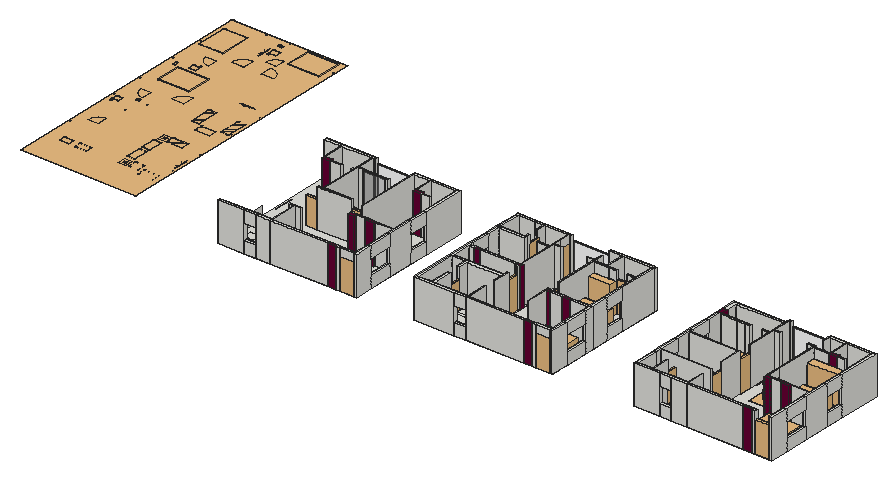
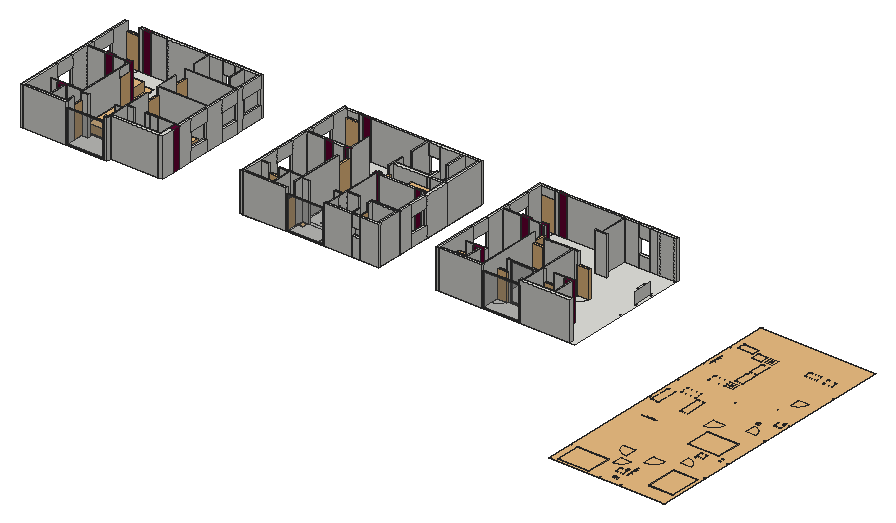
# SketchUp Ruby script. Lengths in inches.
U = 1.inch
M = Sketchup.active_model
def pt(a) = Geom::Point3d.new(a.map { |v| v * U })
def face(e, loops, mat)
  f = e.add_face(loops[0].map { |a| pt(a) })
  loops[1..].each { |l| e.add_face(l.map { |a| pt(a) }).erase! }
  f.material = f.back_material = mat if mat
  f
end
# faces: each face lists its corners as indices into pts; further lists are holes
def faces(e, pts, list, mat = nil) = list.each { |f| face(e, (f[0].is_a?(Array) ? f : [f]).map { |l| l.map { |i| pts[i] } }, mat) }
# xy, xz, yz: faces in a plane at the given z, y or x. An outline is a flat list of corners, or four numbers for a rectangle; further outlines are holes
def ring(l) = l.size == 4 ? [[l[0], l[1]], [l[2], l[1]], [l[2], l[3]], [l[0], l[3]]] : l.each_slice(2).to_a
def flat(e, list, mat, &to3) = list.each { |f| face(e, (f[0].is_a?(Array) ? f : [f]).map { |l| ring(l).map { |u, v| to3.(u, v) } }, mat) }
def xy(e, z, list, mat = nil) = flat(e, list, mat) { |x, y| [x, y, z] }
def xz(e, y, list, mat = nil) = flat(e, list, mat) { |x, z| [x, y, z] }
def yz(e, x, list, mat = nil) = flat(e, list, mat) { |y, z| [x, y, z] }
def lines(e, pts, list) = list.each { |a, b| e.add_line(pt(pts[a]), pt(pts[b])) }
# prism: a flat outline (further loops are holes) pulled along v
def prism(e, loops, v, mat = nil)
  f = face(e, loops, mat); d = Geom::Vector3d.new(v.map { |x| x * U })
  f.pushpull(f.normal.samedirection?(d) ? d.length : -d.length)
end
def box(e, o, s, mat = nil) = prism(e, [[o, [o[0] + s[0], o[1], o[2]], [o[0] + s[0], o[1] + s[1], o[2]], [o[0], o[1] + s[1], o[2]]]], [0, 0, s[2]], mat)
def at(x, y, z, deg = 0) = Geom::Transformation.translation(pt([x, y, z])) * Geom::Transformation.rotation(ORIGIN, Z_AXIS, deg.degrees)
def axes(o, x, y, z) = Geom::Transformation.new([*x, 0, *y, 0, *z, 0, *pt(o).to_a, 1])
def part(name) = M.definitions.add(name)
# library, detail: a bought-in or finely detailed component or shape, given as its bounding box
def library(name, o, s) = part(name).tap { |d| box(d.entities, o, s) }
def detail(e, o, s) = box(e.add_group.entities, o, s)
def put(e, d, t, mat = nil) = e.add_instance(d, t).tap { |i| i.material = mat if mat }
def group(e, t, mat = nil) = e.add_group.tap { |g| g.transformation = t; g.material = mat if mat }.entities
root = M.entities
M.materials.add("L08_Velvet_Rose").color = [102, 0, 51]
M.materials.add("[Color M07]").color = [58, 58, 58]
M.materials.add("[Translucent Glass Gray]3").color = [128, 128, 128]
M.materials["[Translucent Glass Gray]3"].alpha = 0.3
c1 = library("CS300DRT",[0,0,0],[27.18,17.85,30.31])
c2 = library("PINTU+6+YA",[0,-0.6875,0],[35.83,8.07,80.71])
c3 = library("T4592TW1\#2",[64.87,43.1,3.9375],[29.53,8.27,84.64])
c4 = part("WINDOW (1)")
xy(c4.entities,0,[[0,0,59.06,1.97]],"[Color M07]")
xy(c4.entities,1.97,[[1.97,0,57.09,0.98],[1.97,0.98,57.09,1.97]],"[Color M07]")
xy(c4.entities,104.33,[[1.97,0,57.09,0.98],[1.97,0.98,57.09,1.97]],"[Color M07]")
xy(c4.entities,106.3,[[0,0,59.06,1.97]],"[Color M07]")
xz(c4.entities,0,[[[0,0,59.06,106.3],[1.97,1.97,57.09,104.33]]],"[Color M07]")
xz(c4.entities,0.98,[[1.97,1.97,57.09,104.33]],"[Translucent Glass Gray]3")
xz(c4.entities,1.97,[[[0,0,59.06,106.3],[1.97,1.97,57.09,104.33]]],"[Color M07]")
yz(c4.entities,0,[[0,0,1.97,106.3]],"[Color M07]")
yz(c4.entities,1.97,[[0,1.97,0.98,104.33],[0.98,1.97,1.97,104.33]],"[Color M07]")
yz(c4.entities,57.09,[[0,1.97,0.98,104.33],[0.98,1.97,1.97,104.33]],"[Color M07]")
yz(c4.entities,59.06,[[0,0,1.97,106.3]],"[Color M07]")
c5 = part("A$C31921E4A")
p = [[-49.5,1.5,0],[-206.5,1.5,0],[-206.5,10.5,0],[-49.5,10.5,0],[-54.5,119.5,0],[-215.5,119.5,0],
  [-215.5,130.5,0],[-54.5,130.5,0],[206.5,140.5,0],[-54.5,140.5,0],[-54.5,129.5,0],[206.5,129.5,0],
  [215.5,193.5,0],[-215.5,193.5,0],[-215.5,202.5,0],[215.5,202.5,0],[215.5,-202.5,0],[-215.5,-202.5,0],
  [-215.5,-193.5,0],[215.5,-193.5,0],[-215.5,201.5,0],[-206.5,201.5,0],[-206.5,-193.5,0],[-54,201.5,0],
  [-45,201.5,0],[-45,-193.5,0],[-54,-193.5,0],[69,201.5,0],[82.5,201.5,0],[82.5,-54.5,0],
  [69,-54.5,0],[206.5,201.5,0],[215.5,201.5,0],[206.5,-193.5,0],[-206.5,-104.5,0],[-13.5,-104.5,0],
  [-13.5,-113.5,0],[-206.5,-113.5,0],[73.5,-45.5,0],[215.5,-45.5,0],[215.5,-54.5,0],[73.5,-54.5,0]]
lines(c5.entities,p,[[0,1],[1,2],[2,3],[4,5],[5,6],[6,7],[7,4],[8,9],[9,10],[10,11],[11,8],[12,13],
  [13,14],[14,15],[15,12],[16,17],[17,18],[18,19],[19,16],[20,21],[21,22],[22,18],[18,20],[23,24],
  [24,25],[25,26],[26,23],[27,28],[28,29],[29,30],[30,27],[31,32],[32,19],[19,33],[33,31],[34,35],
  [35,36],[36,37],[37,34],[38,39],[39,40],[40,41],[41,38]])
c6 = part("bbd")
p = [[-18,-16,0],[-19,-16,0],[18,-16,0],[19,-16,0],[17.2,19.5,0],[14.88,19.37,0],
  [12.57,19.09,0],[10.29,18.67,0],[8.04,18.1,0],[5.83,17.39,0],[3.67,16.53,0],[1.57,15.54,0],
  [-0.46,14.41,0],[-2.41,13.16,0],[-4.28,11.78,0],[-6.0625,10.28,0],[-7.74,8.68,0],[-9.31,6.96,0],
  [-10.76,5.15,0],[-12.1,3.25,0],[-13.31,1.27,0],[-14.39,-0.78,0],[-15.34,-2.9,0],[-16.14,-5.08,0],
  [-16.81,-7.31,0],[-17.33,-9.57,0],[-17.7,-11.86,0],[-17.93,-14.17,0],[-18,-16.5,0],[19.5,-19.5,0],
  [-19.5,-19.5,0],[17,-16.5,0],[18,-16.5,0],[18,19.5,0],[17.2,-16.5,0],[18,-15.5,0],
  [19.5,-15.5,0],[-17,-19.5,0],[-19.5,-15.5,0],[-18,-15.5,0],[-17,-16.5,0],[17,-19.5,0]]
lines(c6.entities,p,[[0,1],[2,3],[4,5],[5,6],[6,7],[7,8],[8,9],[9,10],[10,11],[11,12],[12,13],[13,14],
  [14,15],[15,16],[16,17],[17,18],[18,19],[19,20],[20,21],[21,22],[22,23],[23,24],[24,25],[25,26],
  [26,27],[27,28],[29,30],[31,32],[32,33],[33,4],[4,34],[34,32],[32,35],[35,36],[36,29],[37,30],
  [30,38],[38,39],[39,28],[28,40],[40,37],[31,41],[41,29]])
c7 = part("dsfdsf")
p = [[0.3125,-5.07,0],[4.47,-11.36,0],[0.3125,5.07,0],[4.83,11.91,0],[-3.07,-16.82,0],[-3.07,17.58,0],
  [-4.83,17.58,0],[-4.83,-16.82,0],[-3.07,-24.19,0],[-3.07,24.19,0],[-1.23,24.19,0],[-1.23,-24.19,0]]
lines(c7.entities,p,[[0,1],[2,3],[4,5],[5,6],[6,7],[7,4],[8,9],[9,10],[10,11],[11,8]])
c8 = library("shower fix",[-3.29,-6,0],[6.58,12,0.01])
c9 = library("column",[-180,-411.5,0],[360,823,0.01])
c10 = library("A$C6B7D3E4E",[-24,-12,0],[48,24,0.01])
c11 = library("A$C5F771FB3",[-34,-12,0],[68,24,0.01])
c12 = part("A$C33265408")
xy(c12.entities,0,[[[-39.82,-20.33,39.82,20.33],[-39.32,-19.83,39.32,19.83]]])
# 48 loose lines left out
c13 = library("A$C6B07298C",[-24,-12,0],[48,24,0.01])
c14 = library("A$C55B13994",[-14,-12,0],[28,24,0.01])
c15 = part("A$C5BA124C3")
p = [[-13,11.96,0],[13,11.96,0],[12,12.96,0],[12,-12.96,0],[13,-11.96,0],[-13,-11.96,0],
  [-12,-12.96,0],[-12,12.96,0],[1.86,-1.16,0],[5.86,-5.16,0],[-1.14,1.84,0],[-5.14,5.84,0],
  [-5.14,-5.16,0],[-1.14,-1.16,0],[1.86,1.84,0],[5.86,5.84,0],[4.86,4.84,0],[4.86,-4.16,0],
  [-4.14,-4.16,0],[-4.14,4.84,0]]
lines(c15.entities,p,[[0,1],[2,3],[4,5],[6,7],[8,9],[10,11],[12,13],[14,15],[14,8],[8,13],[13,10],[10,14],
  [16,17],[17,18],[18,19],[19,16]])
c16 = library("SFFSF",[-14.15,-9.8,0],[28.3,19.6,0.01])
c17 = library("WASH",[-18,-10.5,0],[36,21,0.01])
c18 = library("A$C52781C1C",[-47.97,-37.8,-0.45],[95.94,75.6,0.9])
c19 = library("21''",[-10.5,-8.8125,0],[21,17.625,0.01])
c20 = library("H.F",[-2.42,-4.375,0],[4.84,8.75,0.01])
c21 = library("bed",[-39,-37.8,-0.45],[78,75.6,0.9])
c22 = library("A$C2B1174C3",[-51.98,-32.72,0],[103.96,65.44,0.01])
c23 = library("A$C0C361DB9",[-9.4375,-14.04,0],[18.87,28.08,0.01])
c24 = library("A$C74866C5B",[-64.5625,-43.35,0],[129.125,86.7,0.01])
c25 = library("A$C220A42E9",[-37.46,-31.14,0],[74.92,62.28,0.01])
c26 = library("A$C26C46208",[-9,-9,0],[18,18,0.01])
c27 = part("g+4.dwg")
xy(c27.entities,0,[[797.44,110.07,833.44,110.57],[1450.06,110.07,1486.06,110.57],[2088.94,110.07,2124.94,110.57],[720.78,115.32,721.28,183.32],[2012.28,115.32,2012.78,183.32],
  [1142.78,161.32,1143.28,235.32],[1751.4,161.32,1751.9,235.32],[2434.28,161.32,2434.78,235.32],[720.78,205.32,721.28,266.32],[2012.28,205.32,2012.78,266.32],
  [409.56,285.45,410.06,315.45],[1142.78,317.32,1143.28,377.32],[1751.4,317.32,1751.9,377.32],[2434.28,317.32,2434.78,377.32],[720.78,325.32,721.28,385.32],
  [1329.4,325.32,1329.9,385.32],[2012.28,325.32,2012.78,385.32],[58.56,326.56,59.06,356.56],[409.56,391.15,410.06,421.15],[895.44,445.57,965.44,446.07],
  [129.06,453.76,129.56,483.76],[409.56,489.76,410.06,543.76],[58.56,501.66,59.06,525.66],[1384.02,505.57,1408.02,506.07],[1497.06,505.57,1614.06,506.07],
  [2179.94,505.57,2296.94,506.07],[888.44,507.57,1005.44,508.07],[58.56,594.9,59.06,627.76],[409.56,599.48,410.06,653.48],[58.56,738.47,59.06,756.47],
  [58.56,827.26,59.06,860.13],[409.56,904.75,410.06,937.62],[162.4375,984.51,195.31,985.01],[235.81,984.51,259.81,985.01]])
# 4548 loose lines left out
put(c27.entities,c5,at(1540.56,307.82,0))
put(c27.entities,c6,axes([133.81,792.76,0],[0,0.84615,0],[-0.84615,0,0],[0,0,0.84615]))
put(c27.entities,c6,axes([262.81,893.26,0],[0,-0.84615,0],[-0.84615,0,0],[0,0,0.84615]))
put(c27.entities,c6,axes([108.31,570.77,0],[0.84615,0,0],[0,-0.84615,0],[0,0,0.84615]))
put(c27.entities,c6,axes([103.81,403.26,0],[0.84615,0,0],[0,0.84615,0],[0,0,0.84615]))
put(c27.entities,c7,at(349.43,677.9375,0,-90))
put(c27.entities,c7,at(400.48,353.68,0,180))
put(c27.entities,c7,at(210.48,914.26,0,180))
put(c27.entities,c8,axes([123.31,539.1875,0],[0,-1,0],[-1,0,0],[0,0,1]))
put(c27.entities,c8,axes([81.31,735.76,0],[-1,0,0],[0,1,0],[0,0,1]))
put(c27.entities,c8,axes([226.8,962.26,0],[0,1,0],[1,0,0],[0,0,1]))
put(c27.entities,c9,at(234.31,577.76,0))
put(c27.entities,c10,at(372.31,265.26,0))
put(c27.entities,c11,at(300.12,572.76,0,90))
put(c27.entities,c6,axes([201.3125,843.76,0],[0,-1,0],[-1,0,0],[0,0,1]))
put(c27.entities,c6,at(294.3,843.76,0,-90))
put(c27.entities,c6,axes([201.3125,611.26,0],[0,-1,0],[-1,0,0],[0,0,1]))
put(c27.entities,c11,axes([391.25,572.76,0],[0,1,0],[1,0,0],[0,0,1]))
put(c27.entities,c12,axes([192.88,512.6,0],[-0.97112,0,0],[0,-0.97112,0],[0,0,0.97112]))
put(c27.entities,c13,at(344.54,521.76,0,180))
put(c27.entities,c13,at(287.84,384.83,0,90))
put(c27.entities,c13,axes([331.02,431.26,0],[-1,0,0],[0,1,0],[0,0,1]))
put(c27.entities,c14,at(323.82,281.73,0,180))
put(c27.entities,c15,at(291.26,431.24,0,-90))
put(c27.entities,c15,at(289.25,279.19,0,-90))
put(c27.entities,c13,at(287.84,328.11,0,90))
put(c27.entities,c16,at(111.51,274.6,0,180))
put(c27.entities,c17,axes([164.42,273.14,0],[-0.99391,0,0],[0,0.99391,0],[0,0,0.99391]))
put(c27.entities,c18,axes([144.94,686.18,0.45],[-1,0,0],[0,1,0],[0,0,1]))
put(c27.entities,c19,axes([78.31,513.79,0],[1,0,0],[0,-1,0],[0,0,1]))
put(c27.entities,c20,axes([70.8,498.76,0],[0,-0.68414,0],[-0.68414,0,0],[0,0,0.68414]))
put(c27.entities,c18,axes([102.11,895.53,0.45],[0,-1,0],[-1,0,0],[0,0,1]))
put(c27.entities,c19,axes([130.81,747.74,0],[-1,0,0],[0,1,0],[0,0,1]))
put(c27.entities,c20,axes([138.3125,762.76,0],[0,0.68414,0],[0.68414,0,0],[0,0,0.68414]))
put(c27.entities,c19,axes([235.81,927.79,0],[1,0,0],[0,-1,0],[0,0,1]))
put(c27.entities,c20,axes([228.3,912.76,0],[0,-0.68414,0],[-0.68414,0,0],[0,0,0.68414]))
put(c27.entities,c18,axes([344.96,941.36,0.45],[-1,0,0],[0,1,0],[0,0,1]))
put(c27.entities,c17,axes([2151.05,126.19,0],[-0.99391,0,0],[0,0.99391,0],[0,0,0.99391]))
put(c27.entities,c20,axes([1669.05,451.32,0],[0,-0.68414,0],[-0.68414,0,0],[0,0,0.68414]))
put(c27.entities,c21,at(2103.94,269.52,0.45))
put(c27.entities,c17,axes([1468.17,124.83,0],[-0.99391,0,0],[0,0.99391,0],[0,0,0.99391]))
put(c27.entities,c16,at(1423.21,126.07,0,180))
put(c27.entities,c19,axes([2036.94,450.34,0],[1,0,0],[0,-1,0],[0,0,1]))
put(c27.entities,c20,axes([2029.43,435.32,0],[0,-0.68414,0],[-0.68414,0,0],[0,0,0.68414]))
put(c27.entities,c18,at(1371.86,371.64,0.45,90))
put(c27.entities,c16,at(2102.47,127.66,0,180))
put(c27.entities,c18,axes([1657.77,356.29,0.45],[0,-1,0],[-1,0,0],[0,0,1]))
put(c27.entities,c18,axes([2065.35,388.67,0.45],[-1,0,0],[0,1,0],[0,0,1]))
put(c27.entities,c18,axes([2340.58,353.29,0.45],[0,-1,0],[-1,0,0],[0,0,1]))
put(c27.entities,c19,axes([1676.56,466.34,0],[1,0,0],[0,-1,0],[0,0,1]))
put(c27.entities,c7,axes([2178.77,398.2,0],[1,0,0],[0,-1,0],[0,0,1]))
put(c27.entities,c8,axes([1729.06,495.32,0],[1,0,0],[0,-1,0],[0,0,1]))
put(c27.entities,c8,at(1357.06,495.32,0,180))
put(c27.entities,c19,axes([1637.34,457.32,0],[0,1,0],[1,0,0],[0,0,1]))
put(c27.entities,c20,axes([1652.06,449.81,0],[0.68414,0,0],[0,-0.68414,0],[0,0,0.68414]))
put(c27.entities,c19,axes([2368.94,466.34,0],[1,0,0],[0,-1,0],[0,0,1]))
put(c27.entities,c20,axes([2361.43,451.32,0],[0,-0.68414,0],[-0.68414,0,0],[0,0,0.68414]))
put(c27.entities,c8,axes([2399.5,495.32,0],[1,0,0],[0,-1,0],[0,0,1]))
put(c27.entities,c8,axes([2051.44,481.32,0],[1,0,0],[0,-1,0],[0,0,1]))
put(c27.entities,c6,axes([1023.4375,284.32,0],[0,-0.92308,0],[0.92308,0,0],[0,0,0.92308]))
put(c27.entities,c19,at(2333.94,483.34,0,180))
put(c27.entities,c20,axes([2341.45,498.32,0],[0,0.68414,0],[0.68414,0,0],[0,0,0.68414]))
put(c27.entities,c6,axes([1116.94,126.81,0],[1.10256,0,0],[0,1.10256,0],[0,0,1.10256]))
put(c27.entities,c6,axes([990.44,458.3125,0],[0.76923,0,0],[0,0.76923,0],[0,0,0.76923]))
put(c27.entities,c6,axes([987.44,326.3125,0],[0.92308,0,0],[0,0.92308,0],[0,0,0.92308]))
put(c27.entities,c6,axes([845.44,326.3125,0],[0.92308,0,0],[0,0.92308,0],[0,0,0.92308]))
put(c27.entities,c6,axes([1123.44,452.3125,0],[0.76923,0,0],[0,0.76923,0],[0,0,0.76923]))
put(c27.entities,c6,axes([857.94,442.8125,0],[0.79487,0,0],[0,0.79487,0],[0,0,0.79487]))
put(c27.entities,c6,axes([757.94,183.82,0],[0,0.79487,0],[-0.79487,0,0],[0,0,0.79487]))
put(c27.entities,c6,axes([1725.56,126.81,0],[1.10256,0,0],[0,1.10256,0],[0,0,1.10256]))
put(c27.entities,c6,at(1633.55,285.82,0,-90))
put(c27.entities,c6,axes([1706.06,452.3125,0],[0.76923,0,0],[0,0.76923,0],[0,0,0.76923]))
put(c27.entities,c6,axes([1629.06,486.32,0],[0,0.76923,0],[0.76923,0,0],[0,0,0.76923]))
put(c27.entities,c6,axes([1398.5625,460.32,0],[0,-0.84615,0],[-0.84615,0,0],[0,0,0.84615]))
put(c27.entities,c6,axes([1364.0625,196.32,0],[0,0.92308,0],[-0.92308,0,0],[0,0,0.92308]))
put(c27.entities,c22,at(1542.06,372.7,0,-90))
put(c27.entities,c23,at(1396.02,491.88,0,-90))
put(c27.entities,c23,at(2078.9,477.88,0,-90))
put(c27.entities,c6,axes([2408.44,126.81,0],[1.10256,0,0],[0,1.10256,0],[0,0,1.10256]))
put(c27.entities,c6,axes([2314.9375,284.32,0],[0,-0.92308,0],[0.92308,0,0],[0,0,0.92308]))
put(c27.entities,c24,axes([2365.08,206.97,0],[1,0,0],[0,-1,0],[0,0,1]))
put(c27.entities,c12,at(2234.94,221.71,0,90))
put(c27.entities,c6,axes([2154.44,222.82,0],[0,-1,0],[-1,0,0],[0,0,1]))
put(c27.entities,c6,axes([2154.44,332.82,0],[0,-1,0],[-1,0,0],[0,0,1]))
put(c27.entities,c6,axes([2414.94,452.3125,0],[0.76923,0,0],[0,0.76923,0],[0,0,0.76923]))
put(c27.entities,c6,axes([2311.9375,463.32,0],[0,-0.76923,0],[0.76923,0,0],[0,0,0.76923]))
put(c27.entities,c24,axes([2252.08,366.875,0],[0,-1,0],[-1,0,0],[0,0,1]))
put(c27.entities,c6,axes([2049.44,183.82,0],[0,0.79487,0],[-0.79487,0,0],[0,0,0.79487]))
put(c27.entities,c6,axes([1504.05,483.32,0],[0,0.92308,0],[0.92308,0,0],[0,0,0.92308]))
put(c27.entities,c24,axes([1681.68,206.97,0],[1,0,0],[0,-1,0],[0,0,1]))
put(c27.entities,c7,at(1495.89,153.68,0))
put(c27.entities,c6,axes([1473.0625,284.32,0],[0,-0.92308,0],[-0.92308,0,0],[0,0,0.92308]))
put(c27.entities,c25,axes([1575.53,220.74,0],[1,0,0],[0,-1,0],[0,0,1]))
put(c27.entities,c7,at(1481.23,352.72,0,180))
put(c27.entities,c17,axes([1353.53,124.83,0],[-0.99391,0,0],[0,0.99391,0],[0,0,0.99391]))
put(c27.entities,c26,at(1605.06,457.32,0))
put(c27.entities,c19,axes([1349.56,455.66,0],[1,0,0],[0,-1,0],[0,0,1]))
put(c27.entities,c20,axes([1375.97,446.81,0],[0.68414,0,0],[0,-0.68414,0],[0,0,0.68414]))
c28 = library("Group\#255",[0,0,0],[24.46,94.5,90.01])
c29 = library("Untitled+(2)",[-25.65,-58.99,0],[75.48,89.46,37.24])
c30 = library("michel-club1",[-34.67,-0.85,-0.13],[126.28,91.17,33.41])
xy(root,0,[[692.13,78.48,773.13,88.48],[[773.13,78.48,1071.13,78.48,1071.13,87.48,1114.13,87.48,1114.13,134.48,1123.13,134.48,1123.13,483.48,692.13,483.48,692.13,239.46,701.13,239.48,701.13,239.46,692.13,239.46,692.13,88.48,773.13,88.48],[701.13,172.48,701.14,176.48]],[1071.13,78.48,1114.13,87.48],[1114.13,78.48,1123.13,134.48],[[1300.75,78.48,1731.75,78.48,1731.75,483.48,1589.75,483.48,1589.75,474.48,1472.75,474.48,1472.75,483.48,1300.75,483.48],[1385.75,405.98,1390.75,449.98]],
  [[1984.63,78.48,2414.63,78.48,2414.63,468.48,2272.63,468.48,2272.63,474.48,2149.63,474.48,2149.63,468.48,1984.63,468.48],[1997.61,402.48,1997.63,405.48]],[701.13,172.48,701.14,176.48],[692.13,239.46,701.13,239.46,701.13,239.48],[1997.61,402.48,1997.63,405.48],[1472.75,474.48,1589.75,483.48]])
xy(root,96,[[1071.13,78.48,1114.13,87.48]])
xy(root,120,[[692.13,78.48,773.13,88.48],[1071.13,78.48,1114.13,87.48],[1114.13,78.48,1123.13,134.48]])
xz(root,78.48,[[692.13,0,773.13,120],[1114.13,0,1123.13,120],[1071.13,96,1114.13,120]])
xz(root,87.48,[[1071.13,96,1114.13,120]])
xz(root,88.48,[[692.13,0,701.04,120],[701.04,0,744.13,120],[744.13,0,749.13,120],[749.13,0,773.13,120]])
xz(root,134.48,[[1114.13,0,1123.13,120]])
yz(root,692.13,[[78.48,0,88.48,120]])
yz(root,701.13,[[178.48,0,239.48,36]])
yz(root,773.13,[[78.48,0,88.48,120]])
yz(root,1071.13,[[78.48,96,87.48,120]])
yz(root,1114.13,[[78.48,0,78.48,96,87.48,96,87.48,120,134.48,120,134.48,0],[78.48,96,87.48,120]])
yz(root,1123.13,[[78.48,0,134.48,120]])
g1 = group(root,at(757.13,411.48,0))
box(g1,[0,0,0],[5,63,120])
g2 = group(root,at(757.13,400.48,0),"L08_Velvet_Rose")
prism(g2,[[[25,0,0],[0,0,0],[0,11,0],[5,11,0],[25,11,0],[25,5,0]]],[0,0,120])
put(root,c1,at(762.46,438.7,0))
g3 = group(root,at(706.13,474.48,0))
prism(g3,[[[0,9,0],[158,9,0],[158,0.625,0],[158,0,0],[152,0,0],[147,0,0],[56,0,0],[51,0,0],[0,0,0]]],[0,0,120])
g4 = group(root,at(773.13,78.48,0))
box(g4,[0,0,0],[36,10,36])
box(g4,[0,0,84],[36,10,36])
# 2 loose lines left out
g5 = group(root,at(782.13,400.48,0))
box(g5,[0,0,0],[36,5,120])
put(root,c2,axes([803.13,288.86,0],[1.00475,0,0],[0,-1,0],[0,0,1.04078]))
g6 = group(root,at(809.13,78.48,0))
prism(g6,[[[44,9,0],[44,0,0],[0,0,0],[0,10,0],[44,10,0]]],[0,0,120])
put(root,c3,axes([917.24,442.46,-3.9375],[-1.04987,0,0],[0,-0.83,0],[0,0,1]))
g7 = group(root,at(849.13,400.48,0))
box(g7,[0,0,0],[4,5,120])
g8 = group(root,at(853.13,87.48,0))
prism(g8,[[[0,0,0],[0,1,0],[0,85,0],[4,85,0],[4,0,0]]],[0,0,120])
g9 = group(root,at(853.13,286.48,0))
prism(g9,[[[0,119,0],[0,188,0],[5,188,0],[5,135,0],[5,130,0],[5,0,0],[0,0,0],[0,114,0]]],[0,0,120])
g10 = group(root,at(839.13,172.48,0))
prism(g10,[[[14,0,0],[0,0,0],[0,4,0],[36,4,0],[36,0,0],[18,0,0]]],[0,0,120])
g11 = group(root,at(858.13,416.48,0))
box(g11,[0,0,0],[13,5,120])
g12 = group(root,at(839.13,281.48,0))
prism(g12,[[[0,0,0],[0,5,0],[14,5,0],[19,5,0],[106,5,0],[106,0,0]]],[0,0,120])
g13 = group(root,at(871.13,416.48,0))
xy(g13,0,[[0,0,70,5]])
put(root,c4,axes([871.13,416.87,0],[1.2012,0,0],[0,1.70117,0],[0,0,1.12]))
put(root,c4,axes([863.02,480.73,0],[2,0,0],[0,1,0],[0,0,1]))
g14 = group(root,at(853.13,78.48,0))
prism(g14,[[[180,0,0],[0,0,0],[0,9,0],[4,9,0],[180,9,0]]],[0,0,120])
g15 = group(root,at(941.13,416.48,0))
box(g15,[0,0,0],[10,5,120])
put(root,c2,axes([945.13,288.86,0],[1.00475,0,0],[0,-1,0],[0,0,1.18946]))
put(root,c3,axes([1049.24,459.11,-3.9375],[-1.04987,0,0],[0,-0.83,0],[0,0,1]))
put(root,c2,axes([985.44,275.57,0],[0,-1.01479,0],[-1,0,0],[0,0,1.18946]))
g16 = group(root,at(981.13,235.48,0))
xy(g16,0,[[0,0,5,4]])
g17 = group(root,at(981.13,275.48,0))
box(g17,[0,0,0],[5,199,120])
g18 = group(root,at(981.13,235.48,0))
box(g18,[0,0,0],[5,4,120])
g19 = group(root,at(981.13,224.48,0),"L08_Velvet_Rose")
prism(g19,[[[0,0,0],[0,11,0],[5,11,0],[17,11,0],[17,6,0],[17,0,0]]],[0,0,120])
g20 = group(root,at(998.13,230.48,0))
box(g20,[0,0,0],[35,5,120])
g21 = group(root,at(1033.13,421.48,0))
box(g21,[0,0,0],[5,53,120])
g22 = group(root,at(1033.13,410.48,0),"L08_Velvet_Rose")
prism(g22,[[[0,0,0],[0,11,0],[5,11,0],[25,11,0],[25,5,0],[25,0,0]]],[0,0,120])
g23 = group(root,at(1033.13,78.48,0),"L08_Velvet_Rose")
box(g23,[0,0,0],[26,9,120])
g24 = group(root,at(1033.13,224.48,0),"L08_Velvet_Rose")
prism(g24,[[[0,11,0],[26,11,0],[26,6,0],[26,0,0],[0,0,0],[0,6,0]]],[0,0,120])
g25 = group(root,at(981.13,474.48,0))
prism(g25,[[[0,9,0],[133,9,0],[133,0,0],[57,0,0],[52,0,0],[5,0,0],[0,0,0]]],[0,0,120])
put(root,c1,at(1036.56,438.7,0))
g26 = group(root,at(1059.13,78.48,0))
box(g26,[0,0,0],[12,9,120])
g27 = group(root,at(1058.13,410.48,0))
box(g27,[0,0,0],[26,5,120])
g28 = group(root,at(1059.13,230.48,0))
box(g28,[0,0,0],[55,5,120])
put(root,c2,axes([1071.13,85.86,0],[1.20012,0,0],[0,-1,0],[0,0,1.18946]))
put(root,c3,axes([1182.98,452.46,-4.64],[-1.04987,0,0],[0,-0.83,0],[0,0,1]))
g29 = group(root,at(1114.13,350.48,0))
prism(g29,[[[9,0,0],[0,0,0],[0,124,0],[0,133,0],[9,133,0]]],[0,0,120])
g30 = group(root,at(1114.13,290.48,0))
xy(g30,0,[[0,0,9,60]])
g31 = group(root,at(1114.13,290.48,0))
box(g31,[0,0,0],[9,60,36])
box(g31,[0,0,84],[9,60,36])
# 2 loose lines left out
g32 = group(root,at(1114.13,134.48,0))
box(g32,[0,0,0],[9,74,36])
box(g32,[0,0,84],[9,74,36])
# 2 loose lines left out
g33 = group(root,at(1114.13,208.48,0))
prism(g33,[[[9,82,0],[9,0,0],[0,0,0],[0,22,0],[0,27,0],[0,82,0]]],[0,0,120])
put(root,c27,at(-24.31,-26.84,0))
g34 = group(root,at(1300.75,88.48,0))
box(g34,[0,0,0],[9,128,120])
g35 = group(root,at(1300.75,216.48,0))
prism(g35,[[[9,82,0],[9,75,0],[9,66,0],[9,9.5,0],[9,0,0],[0,0,0],[0,82,0]]],[0,0,120])
g36 = group(root,at(1300.75,399.48,0))
box(g36,[0,0,0],[9,1,120])
g37 = group(root,at(1300.75,358.48,0))
box(g37,[0,0,0],[9,41,120])
g38 = group(root,at(1300.75,298.48,0))
box(g38,[0,0,0],[9,60,36])
box(g38,[0,0,84],[9,60,36])
# 2 loose lines left out
g39 = group(root,at(1300.75,405.98,0))
box(g39,[0,0,0],[9,68.5,120])
g40 = group(root,at(1309.75,405.48,0))
box(g40,[0,0,0],[5,0.5,120])
g41 = group(root,at(1309.75,282.48,0))
box(g41,[0,0,0],[14.5,9,120])
put(root,c1,at(1314.75,418.53,0))
g42 = group(root,at(1309.75,216.48,0))
box(g42,[0,0,0],[39,9.5,120])
g43 = group(root,at(1300.75,474.48,0))
prism(g43,[[[58.97,9,0],[58.97,0,0],[14,0,0],[9,0,0],[0,0,0],[0,9,0]]],[0,0,120])
g44 = group(root,at(1324.25,282.48,0))
box(g44,[0,0,0],[18,9,120],"L08_Velvet_Rose")
g45 = group(root,at(1300.75,399.48,0))
prism(g45,[[[14,6.5,0],[90,6.5,0],[90,0,0],[9,0,0],[9,1,0],[0,1,0],[0,6.5,0],[9,6.5,0],[9,6,0],[14,6,0]]],[0,0,120])
g46 = group(root,at(1348.75,187.48,0))
prism(g46,[[[0,38.5,0],[8.98,38.5,0],[8.98,27.5,0],[8.98,0,0],[0,0,0],[0,29,0]]],[0,0,120])
g47 = group(root,at(1348.75,88.48,0))
box(g47,[0,0,0],[9,63,120])
put(root,c3,axes([1387.42,72.39,-3.91],[0,1.2192,0],[-0.6889,0,0],[0,0,0.99237]))
put(root,c28,axes([1309.75,223.68,0],[0,1,0],[1,0,0],[0,0,1]))
g48 = group(root,at(1300.75,78.48,0))
prism(g48,[[[0,0,0],[0,10,0],[9,10,0],[48,10,0],[57,10,0],[125,10,0],[125,0,0]]],[0,0,120])
g49 = group(root,at(1359.72,474.48,0))
box(g49,[0,0,0],[24,9,60])
box(g49,[0,0,84],[24,9,36])
# 2 loose lines left out
g50 = group(root,at(1385.75,405.98,0))
box(g50,[0,0,0],[5,11,120])
g51 = group(root,at(1385.75,449.98,0))
box(g51,[0,0,0],[5,24.5,120])
put(root,c3,axes([1421.14,344.48,-4.47],[0,1.1176,0],[-0.6889,0,0],[0,0,1.13414]))
g52 = group(root,at(1342.25,282.48,0))
box(g52,[0,0,0],[112,9,120])
g53 = group(root,at(1357.73,214.98,0))
box(g53,[0,0,0],[104.02,11,120])
g54 = group(root,at(1383.72,474.48,0))
prism(g54,[[[0,9,0],[89.03,9,0],[89.03,0,0],[7.03,0,0],[2.03,0,0],[0,0,0]]],[0,0,120])
g55 = group(root,at(1425.75,78.48,0))
prism(g55,[[[0,0,0],[0,10,0],[36,10,0],[36,9,0],[36,0,0]]],[0,0,36])
prism(g55,[[[36,0,84],[0,0,84],[0,10,84],[36,10,84],[36,9,84]]],[0,0,36])
# 2 loose lines left out
g56 = group(root,at(1426.75,399.48,0))
box(g56,[0,0,0],[35,6,120])
put(root,c2,axes([1464.76,474.57,0],[0,-1.01479,0],[-1,0,0],[0,0,1.18946]))
put(root,c2,axes([1466.0625,275.57,0],[0,-1.01479,0],[-1,0,0],[0,0,1.18946]))
g57 = group(root,at(1454.25,281.48,0))
prism(g57,[[[17,0,0],[0,0,0],[0,1,0],[0,10,0],[0,11,0],[7.5,11,0],[12.5,11,0],[17,11,0]]],[0,0,120],"L08_Velvet_Rose")
g58 = group(root,at(1461.75,87.48,0))
prism(g58,[[[0,0,0],[0,1,0],[0,64,0],[5,64,0],[5,0,0]]],[0,0,120])
g59 = group(root,at(1461.75,187.48,0))
prism(g59,[[[0,52,0],[5,52,0],[5,0,0],[0,0,0],[0,27.5,0],[0,38.5,0]]],[0,0,120])
g60 = group(root,at(1461.75,292.48,0))
prism(g60,[[[0,0,0],[0,107,0],[0,113,0],[0,146,0],[5,146,0],[5,129,0],[5,124,0],[5,0,0]]],[0,0,120])
g61 = group(root,at(1461.75,275.48,0))
box(g61,[0,0,0],[5,6,120])
g62 = group(root,at(1461.75,438.48,0))
box(g62,[0,0,96],[5,36,24])
# 3 loose lines left out
g63 = group(root,at(1466.75,416.48,0))
box(g63,[0,0,0],[22.5,5,120])
put(root,c4,axes([1471.64,480.73,0],[2,0,0],[0,1,0],[0,0,1]))
g64 = group(root,at(1461.75,78.48,0))
prism(g64,[[[180,0,0],[0,0,0],[0,9,0],[5,9,0],[180,9,0]]],[0,0,120])
g65 = group(root,at(1567.25,416.48,0))
prism(g65,[[[27.5,0,0],[22.5,0,0],[0,0,0],[0,5,0],[22.5,5,0],[27.5,5,0]]],[0,0,120])
put(root,c2,axes([1594.0625,278.57,0],[0,-1.09597,0],[-1,0,0],[0,0,1.18946]))
g66 = group(root,at(1589.75,159.48,0))
box(g66,[0,0,0],[3.0625,67,120])
g67 = group(root,at(1589.75,235.48,0))
box(g67,[0,0,0],[5,4,120])
g68 = group(root,at(1589.75,421.48,0))
box(g68,[0,0,0],[5,23,120])
g69 = group(root,at(1589.75,278.48,0))
prism(g69,[[[0,0,0],[0,138,0],[5,138,0],[5,137,0],[5,132,0],[5,0,0]]],[0,0,120])
put(root,c3,axes([1625.14,378.57,-3.91],[0,1.016,0],[-0.6889,0,0],[0,0,0.99237]))
g70 = group(root,at(1589.75,226.48,0))
prism(g70,[[[17,0,0],[0,0,0],[0,9,0],[5,9,0],[17,9,0]]],[0,0,120],"L08_Velvet_Rose")
put(root,c1,at(1622.26,419.98,0,90))
g71 = group(root,at(1594.75,410.48,0))
prism(g71,[[[47,0,0],[0,0,0],[0,5,0],[36,5,0],[41,5,0],[47,5,0]]],[0,0,120])
g72 = group(root,at(1606.75,226.48,0))
box(g72,[0,0,0],[35,9,120])
put(root,c28,axes([1594.75,410.48,0],[0,-1,0],[0.75,0,0],[0,0,1]))
g73 = group(root,at(1630.75,415.48,0))
box(g73,[0,0,0],[5,59,120])
put(root,c29,at(1625.13,322.69,0,90))
put(root,c30,axes([1623.03,160.8,0.11],[0.8,0,0],[0,0.696,0],[0,0,0.8]))
g74 = group(root,at(1641.75,410.48,0))
box(g74,[0,0,0],[25,5,120])
g75 = group(root,at(1641.75,226.48,0))
box(g75,[0,0,0],[26,9,120],"L08_Velvet_Rose")
g76 = group(root,at(1641.75,78.48,0))
box(g76,[0,0,0],[26,9,120],"L08_Velvet_Rose")
put(root,c1,at(1641.75,432.47,0))
g77 = group(root,at(1589.75,474.48,0))
prism(g77,[[[0,9,0],[133,9,0],[133,0,0],[46,0,0],[41,0,0],[0,0,0]]],[0,0,120])
g78 = group(root,at(1667.75,78.48,0))
box(g78,[0,0,0],[12,9,120])
put(root,c3,axes([1761.45,452.46,-5.2],[-0.99737,0,0],[0,-0.83,0],[0,0,1.14243]))
g79 = group(root,at(1667.75,226.48,0))
box(g79,[0,0,0],[55,9,120])
put(root,c2,axes([1679.75,85.86,0],[1.20012,0,0],[0,-1,0],[0,0,1.18946]))
g80 = group(root,at(1679.75,78.48,0))
xy(g80,96,[[0,0,43,9]])
xy(g80,120,[[0,0,43,9]])
xz(g80,0,[[0,96,43,120]])
yz(g80,0,[[0,96,9,120]])
yz(g80,43,[[0,96,9,120]])
# 3 loose lines left out
g81 = group(root,at(1696.75,410.48,0))
box(g81,[0,0,0],[26,5,120])
g82 = group(root,at(1722.75,78.48,0))
box(g82,[0,0,0],[9,56,120])
g83 = group(root,at(1722.75,134.48,0))
box(g83,[0,0,0],[9,74,36])
box(g83,[0,0,84],[9,74,36])
# 2 loose lines left out
g84 = group(root,at(1722.75,350.48,0))
prism(g84,[[[9,124,0],[9,0,0],[0,0,0],[0,60,0],[0,65,0],[0,124,0]]],[0,0,120])
g85 = group(root,at(1722.75,208.48,0))
prism(g85,[[[9,27,0],[9,0,0],[0,0,0],[0,18,0],[0,27,0]]],[0,0,120])
g86 = group(root,at(1722.75,474.48,0))
box(g86,[0,0,0],[9,9,120])
g87 = group(root,at(1722.75,235.48,0))
box(g87,[0,0,0],[9,55,120])
g88 = group(root,at(1722.75,290.48,0))
box(g88,[0,0,0],[9,60,36])
box(g88,[0,0,84],[9,60,36])
# 2 loose lines left out
g89 = group(root,at(1983.63,298.48,0))
box(g89,[0,0,0],[9,60,36])
box(g89,[0,0,84],[9,60,36])
# 2 loose lines left out
g90 = group(root,at(1983.63,88.48,0))
box(g90,[0,0,0],[9,68,36])
box(g90,[0,0,84],[9,68,36])
# 2 loose lines left out
g91 = group(root,at(1983.63,156.48,0))
prism(g91,[[[9,0,0],[0,0,0],[0,22,0],[9,22,0],[9,20,0],[9,16,0]]],[0,0,120])
g92 = group(root,at(1983.63,239.48,0))
prism(g92,[[[9,42,0],[9,0,0],[0,0,0],[0,59,0],[9,59,0],[9,47,0]]],[0,0,120])
g93 = group(root,at(1983.63,358.48,0))
box(g93,[0,0,0],[9,44,120])
g94 = group(root,at(1983.63,178.48,0))
box(g94,[0,0,0],[9,61,36])
box(g94,[0,0,84],[9,61,36])
# 2 loose lines left out
g95 = group(root,at(1983.63,402.48,0),"L08_Velvet_Rose")
prism(g95,[[[0,0,0],[0,24,0],[14,24,0],[14,3,0],[13.97,3,0],[13.97,0,0],[9,0,0]]],[0,0,120])
g96 = group(root,at(1983.63,426.48,0))
prism(g96,[[[0,0,0],[0,43,0],[14,43,0],[14,34,0],[14,0,0]]],[0,0,120])
g97 = group(root,at(1997.61,400.48,0))
prism(g97,[[[0.03,5,0],[51.03,5,0],[51.03,0,0],[0,0,0],[0,2,0],[0.03,2,0]]],[0,0,120])
g98 = group(root,at(1983.63,78.48,0))
prism(g98,[[[81,10,0],[81,0,0],[0,0,0],[0,10,0],[9,10,0],[52,10,0],[57,10,0]]],[0,0,120])
put(root,c3,axes([2076.41,73.37,-3.9375],[0,1.04987,0],[-0.83,0,0],[0,0,1]))
put(root,c29,at(2025.79,369.53,0))
g99 = group(root,at(2035.63,88.48,0))
box(g99,[0,0,0],[5,53,120])
g100 = group(root,at(2048.63,400.48,0))
box(g100,[0,0,0],[25,5,120])
g101 = group(root,at(1992.63,281.48,0))
box(g101,[0,0,0],[152,5,120])
put(root,c29,at(2056.8,250.11,0))
g102 = group(root,at(1992.63,172.48,0))
box(g102,[0,0,0],[157,4,120])
g103 = group(root,at(1997.63,460.48,0))
box(g103,[0,0,0],[147,9,120])
g104 = group(root,at(2073.63,400.48,0))
box(g104,[0,0,0],[15,5,120])
g105 = group(root,at(2064.63,78.48,0))
box(g105,[0,0,0],[36,10,36])
box(g105,[0,0,84],[36,10,36])
# 2 loose lines left out
g106 = group(root,at(2100.63,78.48,0))
prism(g106,[[[48.0625,0,0],[0,0,0],[0,10,0],[45.02,10,0],[45.02,9,0],[48.0625,9,0]]],[0,0,120])
g107 = group(root,at(2124.63,400.48,0))
box(g107,[0,0,0],[20,5,120])
put(root,c2,axes([2148.94,215.57,0],[0,-1.09597,0],[-1,0,0],[0,0,1.18946]))
put(root,c2,axes([2148.94,325.48,0],[0,-1.09597,0],[-1,0,0],[0,0,1.18946]))
g108 = group(root,at(2144.63,325.48,0))
prism(g108,[[[0,144,0],[0,149,0],[5,149,0],[5,96,0],[5,91,0],[5,0,0],[0,0,0],[0,75,0],[0,80,0],[0,135,0]]],[0,0,120])
g109 = group(root,at(2144.63,215.48,0))
prism(g109,[[[0,71,0],[5,71,0],[5,0,0],[0,0,0],[0,66,0]]],[0,0,120])
g110 = group(root,at(2145.66,87.48,0))
box(g110,[0,0,0],[3.04,1,120])
g111 = group(root,at(2145.63,87.48,0))
box(g111,[0,0,0],[4,53,120])
g112 = group(root,at(2144.63,474.48,0))
prism(g112,[[[11,9,0],[11,0,0],[5,0,0],[0,0,0],[0,9,0]]],[0,0,120])
g113 = group(root,at(2149.63,416.48,0))
box(g113,[0,0,0],[19.5,5,120])
put(root,c4,axes([2154.52,480.73,0],[2,0,0],[0,1,0],[0,0,1]))
g114 = group(root,at(2155.63,474.48,0))
xy(g114,0,[[0,0,117,9]])
g115 = group(root,at(2148.7,78.48,0))
prism(g115,[[[175.9375,0,0],[0,0,0],[0,9,0],[0.9375,9,0],[123.9375,9,0],[126.9375,9,0],[175.9375,9,0]]],[0,0,120])
put(root,c30,axes([2207.87,328.32,0.11],[0.00599,0.79998,0],[0.69598,-0.00521,0],[0,0,0.8]))
g116 = group(root,at(2253.13,416.48,0))
prism(g116,[[[24.5,5,0],[24.5,0,0],[19.5,0,0],[0,0,0],[0,5,0]]],[0,0,120])
g117 = group(root,at(2272.63,87.48,0))
xy(g117,0,[[0,0,3,22.11]])
g118 = group(root,at(2272.63,152.48,0))
xy(g118,0,[[0,0,3,72]])
put(root,c2,axes([2277.63,275.48,96],[0,-1.01925,0],[-1,0,0],[0,0,-1.18946]))
g119 = group(root,at(2272.63,239.48,0))
box(g119,[0,0,96],[5,36,24])
# 3 loose lines left out
g120 = group(root,at(2272.63,275.48,0))
prism(g120,[[[5,141,0],[5,140.5,0],[5,135.5,0],[5,0,0],[0,0,0],[0,141,0]]],[0,0,120])
g121 = group(root,at(2272.63,451.48,0))
box(g121,[0,0,0],[5,23,120])
g122 = group(root,at(2272.63,235.48,0))
box(g122,[0,0,0],[5,4,120])
put(root,c3,axes([2308.02,355.57,-4.47],[0,1.016,0],[-0.6889,0,0],[0,0,1.13414]))
g123 = group(root,at(2272.63,224.48,0),"L08_Velvet_Rose")
prism(g123,[[[5,11,0],[17,11,0],[17,6,0],[17,0,0],[3,0,0],[0,0,0],[0,11,0]]],[0,0,120])
g124 = group(root,at(2277.63,410.98,0))
box(g124,[0,0,0],[47,5,120])
g125 = group(root,at(2289.63,230.48,0))
box(g125,[0,0,0],[35,5,120])
put(root,c29,at(2308.1,319.33,0,90))
put(root,c28,axes([2277.83,410.48,0],[0,-1,0],[1.035,0,0],[0,0,1]))
g126 = group(root,at(2324.63,421.48,0))
box(g126,[0,0,0],[5,53,120])
g127 = group(root,at(2324.63,410.48,0),"L08_Velvet_Rose")
prism(g127,[[[25,0,0],[0,0,0],[0,0.5,0],[0,5.5,0],[0,11,0],[5,11,0],[25,11,0],[25,5,0]]],[0,0,120])
g128 = group(root,at(2324.63,78.48,0),"L08_Velvet_Rose")
box(g128,[0,0,0],[26,9,120])
g129 = group(root,at(2324.8,224.48,0),"L08_Velvet_Rose")
prism(g129,[[[0,11,0],[25.83,11,0],[25.83,6,0],[25.83,0,0],[0,0,0]]],[0,0,120])
g130 = group(root,at(2272.63,474.48,0))
prism(g130,[[[0,9,0],[133,9,0],[133,0,0],[57,0,0],[52,0,0],[5,0,0],[0,0,0]]],[0,0,120])
put(root,c30,axes([2317.96,158.52,0.11],[0.8,0,0],[0,0.696,0],[0,0,0.8]))
g131 = group(root,at(2350.63,78.48,0))
box(g131,[0,0,0],[12,9,120])
g132 = group(root,at(2349.63,410.48,0))
box(g132,[0,0,0],[26,5,120])
g133 = group(root,at(2350.63,230.48,0))
box(g133,[0,0,0],[55,5,120])
put(root,c2,axes([2362.63,85.86,0],[1.20012,0,0],[0,-1,0],[0,0,1.18946]))
g134 = group(root,at(2405.63,208.48,0))
prism(g134,[[[9,0,0],[0,0,0],[0,22,0],[0,27,0],[0,82,0],[9,82,0]]],[0,0,120])
g135 = group(root,at(2405.63,290.48,0))
box(g135,[0,0,0],[9,60,36])
box(g135,[0,0,84],[9,60,36])
# 2 loose lines left out
g136 = group(root,at(2405.63,78.48,0))
box(g136,[0,0,0],[9,56,120])
g137 = group(root,at(2405.63,134.48,0))
box(g137,[0,0,0],[9,74,36])
box(g137,[0,0,84],[9,74,36])
# 2 loose lines left out
g138 = group(root,at(2405.63,350.48,0))
prism(g138,[[[9,0,0],[0,0,0],[0,124,0],[0,133,0],[9,133,0]]],[0,0,120])
